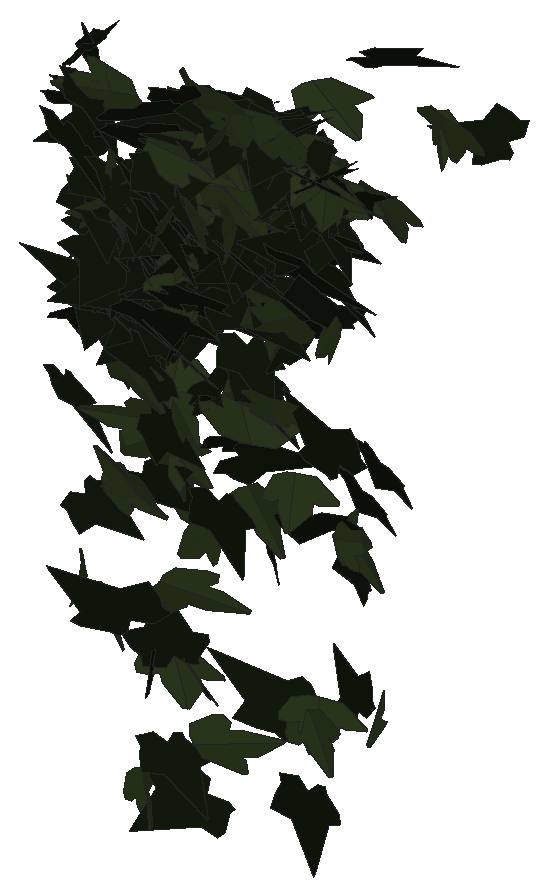
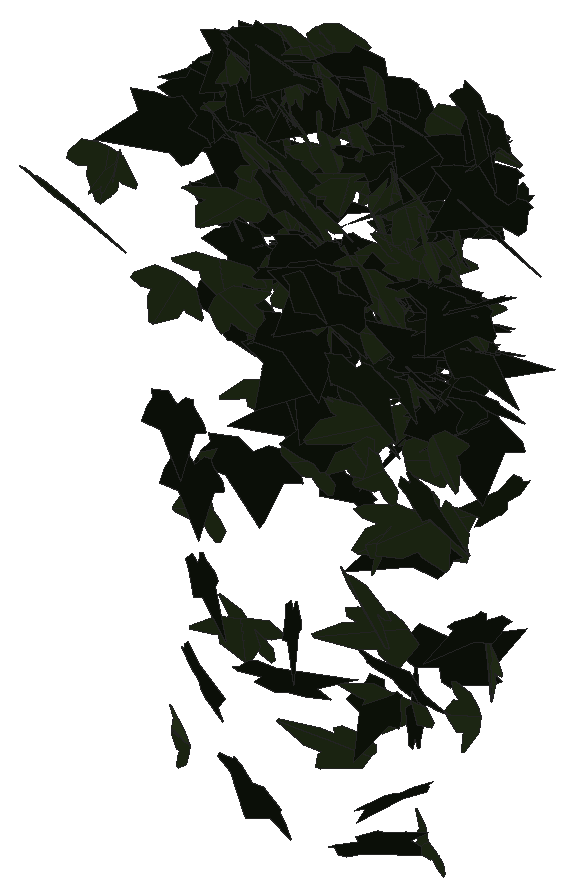
# SketchUp Ruby script. Lengths in millimetres.
U = 1.mm
M = Sketchup.active_model
def pt(a) = Geom::Point3d.new(a.map { |v| v * U })
def face(e, loops, mat)
  f = e.add_face(loops[0].map { |a| pt(a) })
  loops[1..].each { |l| e.add_face(l.map { |a| pt(a) }).erase! }
  f.material = f.back_material = mat if mat
  f
end
# faces: each face lists its corners as indices into pts; further lists are holes
def faces(e, pts, list, mat = nil) = list.each { |f| face(e, (f[0].is_a?(Array) ? f : [f]).map { |l| l.map { |i| pts[i] } }, mat) }
# xy, xz, yz: faces in a plane at the given z, y or x. An outline is a flat list of corners, or four numbers for a rectangle; further outlines are holes
def ring(l) = l.size == 4 ? [[l[0], l[1]], [l[2], l[1]], [l[2], l[3]], [l[0], l[3]]] : l.each_slice(2).to_a
def flat(e, list, mat, &to3) = list.each { |f| face(e, (f[0].is_a?(Array) ? f : [f]).map { |l| ring(l).map { |u, v| to3.(u, v) } }, mat) }
def xy(e, z, list, mat = nil) = flat(e, list, mat) { |x, y| [x, y, z] }
def xz(e, y, list, mat = nil) = flat(e, list, mat) { |x, z| [x, y, z] }
def yz(e, x, list, mat = nil) = flat(e, list, mat) { |y, z| [x, y, z] }
def lines(e, pts, list) = list.each { |a, b| e.add_line(pt(pts[a]), pt(pts[b])) }
# prism: a flat outline (further loops are holes) pulled along v
def prism(e, loops, v, mat = nil)
  f = face(e, loops, mat); d = Geom::Vector3d.new(v.map { |x| x * U })
  f.pushpull(f.normal.samedirection?(d) ? d.length : -d.length)
end
def box(e, o, s, mat = nil) = prism(e, [[o, [o[0] + s[0], o[1], o[2]], [o[0] + s[0], o[1] + s[1], o[2]], [o[0], o[1] + s[1], o[2]]]], [0, 0, s[2]], mat)
def at(x, y, z, deg = 0) = Geom::Transformation.translation(pt([x, y, z])) * Geom::Transformation.rotation(ORIGIN, Z_AXIS, deg.degrees)
def axes(o, x, y, z) = Geom::Transformation.new([*x, 0, *y, 0, *z, 0, *pt(o).to_a, 1])
def part(name) = M.definitions.add(name)
# library, detail: a bought-in or finely detailed component or shape, given as its bounding box
def library(name, o, s) = part(name).tap { |d| box(d.entities, o, s) }
def detail(e, o, s) = box(e.add_group.entities, o, s)
def put(e, d, t, mat = nil) = e.add_instance(d, t).tap { |i| i.material = mat if mat }
def group(e, t, mat = nil) = e.add_group.tap { |g| g.transformation = t; g.material = mat if mat }.entities
root = M.entities
M.materials.add("efeu1").color = [18, 25, 13]
M.materials.add("efeu2").color = [43, 57, 29]
c1 = part("ivyleaf_9")
p = [[39.1,54.8,31.7],[34.5,51.8,30.2],[-5.3,25.2,17.3],[-17.9,28.3,20.9],[-21.6,21.7,17],[-20.2,4.3,5.3],
  [-22.9,-0.3,2.5],[-17.1,-4,-0.6],[-2,-2.1,-1.2],[-0.7,-15.4,-10.1],[16.6,-22.3,-16.7],[21.1,-15.1,-12.5],
  [32.7,-10.7,-11],[46.1,-1.8,-6.6],[30.8,11.2,3.8]]
faces(c1.entities,p,[[0,1,2,3,4,5,6,7,8,9,10,11,12,13,14]],"efeu1")
c2 = part("ivyleaf_10")
p = [[0,12.8,-0.8],[-1.5,51.3,-10.9],[-4.9,51,-11.6],[-13.6,26.5,-7.3],[-13.2,15.9,-4.6],[-21.1,19.3,-7.2],
  [-29.5,16.3,-8.3],[-29.2,8.3,-6.2],[-19.7,-9.8,0.5],[-7.6,-13,4],[1,-12.2,5.8],[-0.4,51.1,-11.1],
  [-1.5,51.1,-10.9],[1,-12.4,5.9],[16.9,-12.4,3.5],[35.1,9.1,-5.1],[35,12.9,-6.1],[20.5,16.4,-4.9],
  [15.8,15,-3.8],[15.3,27.6,-7.1],[12.8,31.3,-7.8]]
faces(c2.entities,p,[[0,1,2,3,4,5,6,7,8,9,10],[11,12,0,13,14,15,16,17,18,19,20]],"efeu2")
put(root,c1,axes([4336.7,826.9,2307.8],[1.64636,0.46181,-0.34816],[-0.57705,-0.1713,-0.98057],[-0.93732,0.91661,-0.00785]))
put(root,c1,axes([4322.9,848,2418.5],[0.66586,-0.92528,0.22306],[0.13804,-0.21105,-0.9892],[1.80618,0.35724,-0.00663]))
put(root,c1,axes([4282.4,847.1,1881.3],[0.46301,0.06255,1.08971],[-2.0489,-0.17041,0.25013],[0.34267,-1.10346,0.02314]))
put(root,c2,axes([4346,845.1,2435.9],[0.56997,-0.94668,0.22063],[0.12351,-0.21088,-0.99292],[1.84587,0.30642,-0.00169]))
put(root,c1,axes([4522.6,843.7,2424.9],[1.00626,-0.4296,0.7182],[1.14423,-0.39598,-0.67945],[1.10798,0.7991,0.04941]))
put(root,c2,axes([4522.3,838.5,2360.9],[-1.30614,-0.1043,0.71245],[-1.34296,-0.09855,-0.69414],[0.27286,-0.98431,-0.00599]))
put(root,c2,axes([4379.4,838.4,2456.6],[-1.04442,0.79665,-0.17631],[0.15381,-0.15836,-0.9671],[-1.54524,-0.55422,0.0229]))
put(root,c2,axes([4531.4,843.4,2142.7],[1.04113,0.86913,-0.2398],[-0.2545,-0.19917,-1.02694],[-1.69696,0.5631,0.00689]))
put(root,c2,axes([4431.2,835.7,2580.5],[0.10633,-0.99685,-0.41769],[-0.09141,0.41555,-0.99815],[2.05498,0.07007,-0.02279]))
put(root,c2,axes([4547.5,850.1,1834.9],[1.39029,-0.29535,0.69025],[1.20953,-0.26951,-0.7879],[0.76078,0.96822,-0.00876]))
put(root,c1,axes([4415.1,850,2074.1],[-0.95308,-0.05464,-0.90576],[1.72252,0.04422,-0.50306],[0.12403,-1.03404,0.02635]))
put(root,c1,axes([4316.3,860.7,2215.4],[0.48235,-0.93383,-0.33429],[0.2204,-0.31481,0.96721],[-1.8748,-0.27727,0.0277]))
put(root,c1,axes([4184.4,857.9,2481.5],[0.57821,-0.94323,0.32201],[0.18852,-0.3064,-0.99095],[1.88748,0.31955,0.00033]))
put(root,c2,axes([4441.8,834.8,2450.9],[0.64325,-0.75033,-0.66937],[-0.24935,0.66729,-0.81415],[1.89737,0.34207,0.11993]))
put(root,c2,axes([4259.2,852.9,2048.7],[0.03094,-0.11636,1.02492],[1.92704,-0.19391,-0.03808],[0.37482,1.00654,0.11115]))
put(root,c2,axes([4300.1,842.9,2051.3],[-1.15507,0.33695,-0.68674],[-1.14276,0.33329,0.69418],[0.902,0.85374,0.00005]))
put(root,c1,axes([4334.4,853.2,2487.2],[-0.02576,-0.98001,-0.37608],[-0.01723,0.37621,-0.98001],[1.9977,-0.00939,-0.0133]))
put(root,c1,axes([4357.7,839.3,2331.6],[1.83908,0.03973,0.39257],[0.74506,0.03333,-0.967],[-0.09391,1.04248,0.01596]))
put(root,c2,axes([4444.3,839.5,2600.2],[1.07842,-0.10726,-0.85706],[-1.25103,0.6114,-0.51111],[1.06642,0.82572,0.26711]))
put(root,c2,axes([4299.9,861.3,2139.4],[-0.18622,-0.05734,-0.98275],[-1.58696,-0.52011,0.11337],[-0.99586,0.83955,0.00311]))
put(root,c2,axes([4269.8,852.1,2562.1],[-0.62328,-0.02674,0.99814],[-1.80991,-0.31185,-0.32037],[0.57928,-1.00314,0.07299]))
put(root,c1,axes([4596,837.9,2199],[0.10505,0.013,1.05977],[-1.01079,0.91869,0.01639],[-1.74558,-0.5312,0.05429]))
put(root,c2,axes([4502.7,850.6,2587.7],[-1.6085,0.20624,0.52283],[-1.06539,-0.22451,-0.81634],[-0.09559,-0.96811,0.30069]))
put(root,c1,axes([4300.5,854.9,2270.2],[1.37428,-0.63325,0.29637],[0.42664,-0.19388,-0.96043],[1.26042,0.75608,0.00195]))
put(root,c2,axes([4287.5,863,1665.3],[0.94142,-0.46315,0.75785],[1.13813,-0.4677,-0.67614],[1.2498,0.77478,0.04488]))
put(root,c2,axes([4274.9,854,2206.2],[-1.31652,0.30846,-0.60263],[0.95598,-0.34379,-0.75254],[-0.86383,-0.85057,0.08563]))
put(root,c1,axes([4432.5,855.7,2404],[1.21331,-0.69179,0.2791],[0.56068,-0.10382,-0.93022],[1.30432,0.68814,0.14024]))
put(root,c1,axes([4212.2,863.4,2545.1],[0.3497,-0.99056,0.1031],[0.0191,-0.103,-1.00742],[1.89533,0.1838,-0.00887]))
put(root,c2,axes([4338.7,848,2510.1],[0.32722,0.10037,1.09442],[1.953,0.38191,-0.19624],[-0.74881,1.03993,-0.03357]))
put(root,c1,axes([4307.3,838.8,2532.6],[1.37502,0.84775,-0.11153],[-0.14426,-0.08193,-1.11384],[-1.62094,0.72643,0.00452]))
put(root,c2,axes([4221.6,840.6,1918],[0.25639,-0.64866,-0.7827],[-0.22404,0.77428,-0.66194],[1.92169,0.17682,0.02726]))
put(root,c1,axes([4305.4,836.8,2558.9],[1.18281,0.92076,0.13104],[0.13898,0.10881,-1.11087],[-1.76458,0.62576,0.00034]))
put(root,c1,axes([4294.3,863.2,2433.9],[-1.39195,-0.05491,-0.66628],[1.27237,-0.06017,-0.72889],[-0.00014,-0.98753,0.08146]))
put(root,c1,axes([4256,858.1,2450.2],[-0.57577,-0.80343,-0.59031],[0.52539,0.52526,-0.85637],[1.82326,-0.40507,0.06036]))
put(root,c1,axes([4536.2,847.6,2451.3],[-1.14206,0.72192,0.3168],[-0.42433,0.22648,-0.93841],[-1.43917,-0.63965,0.02529]))
put(root,c1,axes([4458.1,854.8,2405.9],[-1.5319,0.56318,-0.06811],[0.12643,-0.02384,-0.98219],[-1.07222,-0.80743,-0.01851]))
put(root,c1,axes([4258.6,872.3,2295.8],[-1.38533,-0.32585,0.53966],[-0.69948,-0.45038,-0.76767],[0.97479,-0.78627,0.21608]))
put(root,c2,axes([4449.9,865.5,2085.1],[1.27779,-0.27247,0.87737],[1.55773,-0.31617,-0.72451],[0.79415,1.05858,0.00944]))
put(root,c1,axes([4539.3,862.8,2356.5],[1.49916,0.20273,0.63781],[-1.20895,-0.08367,0.8111],[0.40103,-1.01009,0.06083]))
put(root,c2,axes([4425.1,854,2545.5],[1.82145,0.15262,0.27487],[0.44638,0.23996,-0.94984],[-0.39849,0.96639,0.19244]))
put(root,c1,axes([4322.2,846.9,2158.3],[0.88214,-0.57586,-0.8525],[-0.84132,0.73282,-0.73536],[1.76798,0.63605,0.07542]))
put(root,c1,axes([4485.1,875.7,2573.5],[-1.14912,-0.78567,0.20996],[0.04773,-0.27937,-0.97327],[1.54703,-0.57497,0.18599]))
put(root,c1,axes([4482.1,868.9,2549.2],[-1.38832,-0.60821,-0.28835],[0.52732,0.11619,-0.946],[1.16749,-0.77574,0.08439]))
put(root,c2,axes([4348.4,862.3,2328.7],[1.79236,-0.18503,0.16172],[0.29742,-0.04339,-0.95969],[0.36094,0.95456,-0.01228]))
put(root,c1,axes([4389,861.7,2551.6],[-1.69256,0.28049,0.42264],[-0.81052,0.05053,-0.92966],[-0.52443,-0.98335,0.07278]))
put(root,c2,axes([4451.8,856.8,2181.7],[2.06992,0.29269,0.18353],[-0.33795,-0.04641,1.12629],[0.564,-1.102,0.00131]))
put(root,c2,axes([4459.1,864.3,2581.5],[-0.88613,-0.87306,0.18737],[-0.15134,-0.16994,-0.98941],[1.6927,-0.47225,0.00963]))
put(root,c2,axes([4272.9,849.8,2386.9],[-0.79526,0.74822,0.45618],[-0.58732,0.34737,-0.85243],[-1.56098,-0.51189,0.08832]))
put(root,c1,axes([4422.1,873.8,2573.6],[-1.2461,-0.77245,-0.08162],[0.22853,0.00481,-1.00875],[1.46054,-0.65979,0.0882]))
put(root,c1,axes([4299.4,873.3,1802.4],[0.15312,0.38579,0.9606],[-0.56981,-0.91364,0.39201],[1.88593,-0.30737,0.04045]))
put(root,c2,axes([4485.1,859.4,2224.9],[-1.8026,-0.23174,0.09144],[-0.16487,-0.03069,-0.97504],[0.44456,-0.95105,0.00919]))
put(root,c1,axes([4245.2,875.6,2329],[-1.18718,-0.71816,0.13],[-0.17645,-0.09165,-0.95119],[1.37775,-0.63056,-0.0098]))
put(root,c1,axes([4320.1,881.8,2390.7],[-1.36391,-0.52105,0.38349],[-0.152,-0.49666,-0.82406],[1.22187,-0.6434,0.32556]))
put(root,c1,axes([4252.3,863.5,2282.6],[-0.35165,0.08846,0.99512],[-1.77846,0.34265,-0.20396],[-0.67253,-0.95236,0.01905]))
put(root,c2,axes([4547.3,865,1846.2],[1.49454,0.64052,-0.09761],[-0.14355,-0.06196,-1.01338],[-1.22474,0.78889,-0.00034]))
put(root,c1,axes([4432,862,2346.9],[-0.01882,-0.55376,-0.81589],[0.93603,0.70442,-0.48407],[1.62658,-0.41177,0.26912]))
put(root,c2,axes([4540.3,881.4,2542.4],[-0.81762,-0.52454,0.73994],[0.08448,-0.82993,-0.56256],[1.72414,-0.20808,0.37846]))
put(root,c1,axes([4438.6,876.6,2416.2],[-1.1189,-0.78595,-0.12915],[0.14919,0.10264,-0.98151],[1.50853,-0.59311,0.00128]))
put(root,c2,axes([4570.4,863,2350.9],[0.89486,-0.86818,-0.31057],[-0.21441,0.29192,-0.98659],[1.74172,0.48199,0.03811]))
put(root,c1,axes([4357.2,842.6,2262.5],[0.16497,0.29612,1.08571],[0.45443,1.0593,-0.30797],[-2.09304,0.25333,0.01871]))
put(root,c1,axes([4365.8,866.2,2343.6],[-1.62969,0.46454,0.01801],[-0.02518,0.01337,-0.97417],[-0.88443,-0.85637,-0.00545]))
put(root,c2,axes([4319.4,872.4,2480.7],[1.39844,-0.64544,0.17662],[0.25266,-0.11649,-0.97801],[1.24825,0.74668,0.00009]))
put(root,c2,axes([4352.6,858.4,2171.3],[-0.25318,0.94291,0.28828],[-0.14601,0.28011,-0.95159],[-1.87085,-0.14946,0.03526]))
put(root,c1,axes([4324.8,871.5,1717],[0.20585,-0.95763,-0.34904],[-0.01574,0.35016,-0.96327],[1.93978,0.10446,0.02922]))
put(root,c2,axes([4236.4,876.2,2454.4],[0.56437,-0.85145,0.44654],[0.84624,-0.29287,-0.85371],[1.62238,0.44895,0.28996]))
put(root,c1,axes([4352.8,867.3,2510.2],[1.54418,-0.57448,-0.09652],[-0.13237,0.06878,-0.99402],[1.10074,0.81418,0.01587]))
put(root,c1,axes([4524.8,863.1,2534.4],[1.66482,-0.32857,0.32868],[0.7278,0.11076,-0.90701],[0.50266,0.92787,0.22466]))
put(root,c1,axes([4170.7,877.3,2138.1],[0.75934,-0.90696,0.08901],[0.05374,-0.08481,-0.9908],[1.73358,0.3999,-0.00827]))
put(root,c2,axes([4421.3,868.4,2471.1],[-1.69603,-0.15315,-0.37504],[0.74793,-0.10685,-0.89016],[0.18715,-0.96092,0.15876]))
put(root,c2,axes([4314.3,863.7,2444],[-1.59618,0.49111,0.21229],[-0.39179,0.06814,-0.97089],[-0.93988,-0.86245,0.04418]))
put(root,c1,axes([4360.1,882.7,2513.3],[-1.08671,-0.82078,-0.06248],[0.19118,0.006,-0.99674],[1.55492,-0.57437,0.07888]))
put(root,c1,axes([4411.1,866.2,2357.1],[0.25027,-0.39991,-0.89106],[1.21835,0.71433,-0.22612],[1.40386,-0.54864,0.35509]))
put(root,c1,axes([4356.7,854.8,2591.6],[1.49809,0.65891,0.10361],[0.16983,0.0548,-1.02642],[-1.25804,0.79204,-0.01518]))
put(root,c1,axes([4271.9,878,2444.5],[0.90465,-0.87456,0.13595],[0.18084,-0.103,-0.99481],[1.67472,0.48354,0.03398]))
put(root,c2,axes([4462.1,876.5,2565.8],[-0.08543,-0.98427,0.20514],[0.08743,-0.20714,-0.9838],[1.91151,-0.03451,0.05417]))
put(root,c2,axes([4548,873.7,2527.9],[1.90208,-0.12496,0.14333],[0.26808,-0.02865,-1.00714],[0.24313,1.00923,-0.01084]))
put(root,c1,axes([4300.4,878.4,2255.6],[-1.87327,-0.05458,-0.09049],[0.17128,0.01136,-0.98577],[0.10541,-0.98836,-0.00633]))
put(root,c2,axes([4335.9,873.3,2470.5],[-0.2608,0.94177,-0.27405],[-0.1007,-0.28341,-0.94747],[-1.86401,-0.11646,0.08953]))
put(root,c1,axes([4510.4,889.3,2509.5],[-0.42697,-0.88497,0.38336],[0.02153,-0.39598,-0.90749],[1.83539,-0.20123,0.09983]))
put(root,c1,axes([4552.8,850.6,2542.6],[0.73024,0.61781,0.68585],[0.54545,0.62631,-0.72451],[-1.67,0.47472,0.06327]))
put(root,c1,axes([4340.4,859.3,1850.3],[-1.7666,0.41046,-0.14762],[-0.27976,0.03244,1.0145],[0.78161,0.93933,0.02947]))
put(root,c2,axes([4329.8,872.5,1831.9],[1.82053,0.23973,0.27],[0.49217,0.07869,-0.98606],[-0.47957,0.99082,0.01298]))
put(root,c1,axes([4395.9,876.1,2372.1],[0.15595,0.35207,-0.91618],[-1.01845,-0.75468,-0.33787],[-1.56594,0.52589,0.1285]))
put(root,c2,axes([4528.2,882.9,2568.9],[-0.52874,-0.86274,0.42387],[0.18945,-0.46466,-0.88053],[1.81959,-0.20232,0.21485]))
put(root,c1,axes([4202.8,863,2541.9],[1.88988,0.18995,0.03398],[0.0688,-0.00816,-1.0109],[-0.36075,0.99355,-0.0148]))
put(root,c1,axes([4525.8,878.4,2577.8],[-1.88157,0.10593,-0.05742],[0.11395,0.02006,-0.99395],[-0.19899,-0.9901,-0.02628]))
put(root,c1,axes([4357.5,892.7,1655.3],[-1.37979,-0.66511,0.54562],[-0.73639,-0.38518,-0.98366],[1.46232,-0.82154,0.01947]))
put(root,c1,axes([4462.2,891.5,2369.1],[-0.77523,-0.82366,0.36064],[-0.03271,-0.38872,-0.9072],[1.71097,-0.38063,0.14606]))
put(root,c2,axes([4320.5,877.7,2371.1],[1.62868,-0.40605,0.19881],[0.3744,-0.04877,-0.94639],[0.77473,0.87719,0.03942]))
put(root,c1,axes([4532.3,886,2471.8],[-1.44187,-0.555,-0.33157],[0.61868,0.1145,-0.93442],[1.06357,-0.81902,0.09405]))
put(root,c2,axes([4391.3,867.3,1746.9],[0.65297,0.03843,-0.97279],[1.78371,0.26609,0.34106],[0.50143,-0.9966,0.05355]))
put(root,c2,axes([4384.9,879.9,2538.7],[1.29361,-0.73774,0.09596],[0.23957,-0.01406,-0.99971],[1.39547,0.6863,0.08267]))
put(root,c2,axes([4418.6,876.4,2568.2],[1.23058,-0.77001,-0.12744],[0.09858,0.20746,-0.99071],[1.48214,0.62552,0.17171]))
put(root,c2,axes([4362,871.7,2589.9],[-1.37458,0.69827,0.15516],[-0.3317,0.04206,-1.00058],[-1.32033,-0.73753,0.08984]))
put(root,c1,axes([4215.1,856.3,2596.1],[0.18988,0.79581,0.6446],[0.18008,0.63772,-0.80196],[-1.94077,0.13703,-0.01135]))
put(root,c1,axes([4541.5,890.4,2478.7],[0.24706,-0.96576,0.16948],[-0.00151,-0.17106,-0.97416],[1.86611,0.12772,-0.02322]))
put(root,c1,axes([4437.6,883.4,2236.2],[0.49656,-0.95777,-0.20472],[0.04968,0.21859,-0.98937],[1.86335,0.24941,0.08093]))
put(root,c2,axes([4210.1,889.1,1864.4],[-0.6362,0.62383,-0.84867],[0.75258,-0.75093,-0.70773],[-1.85797,-0.51778,0.00393]))
put(root,c1,axes([4443.7,858.5,2143.4],[0.19481,0.39849,-0.95616],[0.11259,0.957,0.40517],[1.96826,-0.09418,0.07146]))
put(root,c2,axes([4483.5,887.2,2324.6],[-0.27053,-0.9101,0.34763],[0.19256,-0.3632,-0.90949],[1.84413,-0.09559,0.14596]))
put(root,c2,axes([4452.5,890.7,2524.6],[0.96675,-0.56051,0.63878],[0.81475,-0.4741,-0.75643],[1.39719,0.66429,-0.00088]))
put(root,c2,axes([4261.3,883,2422.2],[1.24943,-0.72856,0.031],[0.08612,-0.00094,-0.98015],[1.38518,0.65722,0.03297]))
put(root,c1,axes([4491,877.1,2557.6],[1.65215,-0.46822,-0.09834],[-0.15109,0.05995,-0.98619],[0.89793,0.87158,0.015]))
put(root,c1,axes([4426.6,887.1,2266.7],[0.07041,-0.95839,-0.1884],[-0.04939,0.1875,-0.95892],[1.85825,0.0413,-0.01835]))
put(root,c1,axes([4537.6,887.3,2413.8],[0.88405,-0.87812,0.05848],[0.08537,-0.04242,-0.99321],[1.67277,0.46625,0.01978]))
put(root,c2,axes([4310.9,883.1,2399.3],[1.69708,0.3146,-0.20741],[-0.37969,-0.05787,-0.9455],[-0.6084,0.91367,0.01153]))
put(root,c1,axes([4225.3,865.3,2581.9],[0.14706,0.24441,-0.99432],[-1.8605,0.31424,0.00128],[0.5797,0.94652,0.25633]))
put(root,c1,axes([4246.8,886,2413.9],[1.10153,-0.79009,-0.00887],[0.0066,0.01353,-0.97934],[1.50377,0.57869,0.01079]))
put(root,c1,axes([4333.8,899.5,2276.1],[-0.41853,-0.8844,0.3419],[-0.01455,-0.34931,-0.90849],[1.80454,-0.20794,0.07197]))
put(root,c1,axes([4215.7,892.6,2264.4],[-1.52602,-0.36143,-0.36519],[0.71846,0.04477,-0.87315],[0.66337,-0.87993,0.10558]))
put(root,c2,axes([4254.8,888.2,2406.7],[-0.53918,-0.90798,0.17177],[0.12694,-0.19929,-0.94341],[1.75413,-0.26467,0.12107]))
put(root,c2,axes([4476.7,888.8,2541.2],[0.74188,-0.90322,0.13286],[0.11564,-0.11848,-0.98371],[1.73365,0.39442,0.00876]))
put(root,c1,axes([4307.5,891.3,2351.9],[-1.79593,-0.06464,-0.21251],[0.40838,-0.02559,-0.94503],[0.10925,-0.96693,0.03922]))
put(root,c1,axes([4504.7,868.2,2584.1],[0.27662,0.99306,0.14389],[0.08011,0.13923,-1.00341],[-1.90804,0.14981,-0.02127]))
put(root,c1,axes([4423.7,877.1,2547.8],[1.80654,-0.21762,-0.23757],[-0.43238,0.07196,-0.97366],[0.43476,0.97584,0.01882]))
put(root,c2,axes([4485.3,889.8,2439.7],[1.28468,-0.67362,0.27035],[0.46527,-0.13663,-0.95082],[1.30071,0.71418,0.0731]))
put(root,c1,axes([4239.5,895.6,2349.9],[-1.41722,-0.60263,-0.04579],[0.08467,0.0178,-0.95784],[1.1471,-0.74585,0.01413]))
put(root,c1,axes([4392.9,875.7,2203.2],[-0.89263,0.83705,0.12655],[-0.13675,0.10479,-0.95943],[-1.60537,-0.47435,0.01136]))
put(root,c1,axes([4544,874.7,2459.8],[1.40567,0.50277,-0.43038],[-0.73149,-0.19917,-0.89225],[-1.02541,0.8313,0.04652]))
put(root,c1,axes([4219.2,885.2,2489],[-1.6656,0.48207,0.03648],[-0.05871,0.0196,-0.99914],[-0.91822,-0.8757,-0.00228]))
put(root,c1,axes([4530.8,869.6,2548],[-0.44916,0.73124,0.63325],[-0.51019,0.57686,-0.76603],[-1.76891,-0.35206,0.06014]))
put(root,c1,axes([4296,881.9,2473.2],[0.97431,-0.72194,-0.47513],[-0.07203,0.53297,-0.85061],[1.64329,0.4514,0.24442]))
put(root,c1,axes([4340.9,876.2,1834.4],[1.43036,-0.19926,-0.68491],[-1.20194,0.27667,-0.77347],[0.63115,0.97847,0.07922]))
put(root,c2,axes([4540.2,888.3,2503.4],[1.23302,0.7063,-0.25248],[-0.42752,-0.13561,-0.95577],[-1.36202,0.68197,0.07144]))
put(root,c2,axes([4292.6,893,2353.3],[-0.3319,0.78244,-0.53018],[0.19673,-0.52011,-0.80157],[-1.78801,-0.20247,0.01022]))
put(root,c1,axes([4411,874.2,2195.2],[1.43513,0.60791,-0.08571],[-0.1113,-0.06402,-0.9685],[-1.1631,0.75621,-0.01308]))
put(root,c1,axes([4206.1,888,2253.9],[1.47083,-0.60709,0.0565],[0.07802,-0.03928,-0.98274],[1.15778,0.77389,-0.00556]))
put(root,c1,axes([4522.4,878.6,2517.7],[-0.37238,0.96299,-0.1223],[0.03004,-0.12158,-0.98263],[-1.84725,-0.1961,0.00867]))
put(root,c2,axes([4293.3,888.3,2449.4],[-0.46612,-0.9614,-0.02234],[-0.01017,0.02441,-0.99204],[1.8302,-0.24471,-0.0112]))
put(root,c1,axes([4200.3,899.5,2380.4],[-0.32394,-0.95833,0.01524],[0.03539,-0.01877,-0.97309],[1.82378,-0.16985,0.02159]))
put(root,c2,axes([4399.6,892.4,2491.7],[0.25391,-0.96725,-0.13885],[0.03231,-0.13782,0.97641],[-1.85947,-0.13448,-0.00199]))
put(root,c1,axes([4537.7,877.5,2544.1],[1.72379,0.04013,-0.61368],[-1.17012,0.08494,-0.90186],[0.0277,1.09075,0.09281]))
put(root,c1,axes([4493.7,890.1,1811.9],[-1.6303,-0.51484,-0.34167],[-0.56032,-0.1734,0.99942],[-1.03391,0.90579,-0.00287]))
put(root,c2,axes([4213.6,895.2,2370.3],[-0.62713,-0.86435,0.28217],[-0.06449,-0.28825,-0.92253],[1.72926,-0.32421,0.06793]))
put(root,c1,axes([4220.1,906.7,2280.1],[0.52651,-0.27868,-0.87738],[1.18957,-0.61575,0.39266],[-1.28631,-0.68351,0.004]))
put(root,c1,axes([4395.8,887,2129.2],[1.26068,0.73295,0.16831],[-0.21956,-0.1226,0.98792],[1.41432,-0.67236,0.00334]))
put(root,c1,axes([4240.9,904.4,2307],[-1.0998,-0.7499,0.17358],[-0.19578,-0.13987,-0.94671],[1.4518,-0.58694,0.00383]))
put(root,c2,axes([4444.6,889.4,2412],[1.61031,-0.36772,-0.35356],[-0.59114,0.17182,-0.92202],[0.77013,0.90077,0.03155]))
put(root,c2,axes([4333.3,898.2,2445.1],[0.86615,-0.80039,0.327],[0.31194,-0.28297,-0.92073],[1.6157,0.48371,0.00246]))
put(root,c1,axes([4252.2,894.4,2353.6],[0.95858,-0.8208,-0.00799],[0.08908,0.03807,-0.96116],[1.55968,0.50229,0.0598]))
put(root,c2,axes([4255.7,894.5,2408.6],[0.72014,-0.88399,-0.20248],[0.1248,-0.19215,0.96145],[-1.72146,-0.38373,-0.015]))
put(root,c2,axes([4319.5,893.8,2201.4],[0.9224,0.78049,-0.29783],[-0.31397,-0.24813,-0.91868],[-1.55859,0.51189,0.0088]))
put(root,c2,axes([4383.4,889.2,2464.8],[0.69026,0.90878,-0.04945],[-0.05156,-0.04243,-0.97843],[-1.73138,0.36357,0.00943]))
put(root,c1,axes([4179.6,876.4,2516.8],[1.63682,0.47043,0.25534],[0.37972,0.16666,-0.97907],[-0.94529,0.88152,0.04884]))
put(root,c2,axes([4328.7,881.4,1923.6],[-0.79422,-0.16365,-0.98224],[1.72042,0.38442,-0.4481],[0.79486,-0.99557,-0.01157]))
put(root,c1,axes([4327.7,900,2349.9],[0.9793,0.37373,0.736],[-1.11077,-0.44861,0.63582],[1.11097,-0.77796,-0.01307]))
put(root,c1,axes([4505.9,876.8,2337.1],[1.10843,0.79379,0.0726],[0.0642,0.06528,-0.98447],[-1.5157,0.58327,0.01139]))
put(root,c2,axes([4314.1,899.9,2339.7],[0.17693,-0.93451,0.23239],[-0.01295,-0.2341,-0.93867],[1.83268,0.08857,-0.02907]))
put(root,c1,axes([4517.2,884,2078.2],[0.90443,0.81082,-0.33488],[-0.40556,-0.26276,-0.93859],[-1.61958,0.51859,0.04803]))
put(root,c1,axes([4320.8,904.6,2280.2],[-1.55102,-0.45221,-0.25531],[0.53872,0.01149,-0.92389],[0.8286,-0.85393,0.12277]))
put(root,c1,axes([4286.2,902.6,2313.6],[0.68531,-0.89443,0.10005],[0.09176,-0.08844,-0.96412],[1.71043,0.36311,0.01164]))
put(root,c1,axes([4292.3,905.3,2262.6],[-0.71514,-0.88439,-0.09622],[0.04585,0.0943,-0.96079],[1.69248,-0.37624,-0.01463]))
put(root,c1,axes([4552.7,884.8,2479.6],[-0.98377,0.80965,0.27333],[-0.27993,0.23038,-0.96058],[-1.60208,-0.53742,0]))
put(root,c2,axes([4272.7,904.4,2253.5],[1.14496,-0.3423,0.67466],[1.10961,-0.33951,-0.69215],[0.91751,0.83775,-0.00484]))
put(root,c1,axes([4280.6,884.4,2050],[-0.0227,-0.22479,-0.93849],[0.45661,0.90841,-0.22063],[1.77899,-0.23603,0.04465]))
put(root,c2,axes([4357.4,898.2,2373.4],[-1.04902,-0.8014,0.07954],[0.09738,-0.13104,-0.96571],[1.52962,-0.54126,0.11603]))
put(root,c2,axes([4361.8,899.3,2373.9],[1.32777,-0.67705,0.08199],[0.2574,0.02239,-0.96594],[1.27219,0.7021,0.10986]))
put(root,c1,axes([4213.9,906.9,2219.8],[-0.06329,-0.9598,-0.02296],[-0.02459,0.02342,-0.96028],[1.82704,-0.03293,-0.01372]))
put(root,c2,axes([4483.6,890.4,2447.6],[-0.35193,-0.85888,0.45642],[0.16563,0.44813,0.87852],[-1.84368,0.20421,-0.0082]))
put(root,c1,axes([4243.7,902.4,2388.2],[-0.89815,-0.66497,-0.52291],[0.57627,0.42633,-0.81541],[1.50334,-0.5607,0.00016]))
put(root,c1,axes([4477.8,877.2,2589.4],[1.049,0.72166,0.43785],[-0.05314,0.53823,-0.85196],[-1.60562,0.45367,0.31426]))
put(root,c1,axes([4210.9,899.7,2331],[-0.63091,0.76712,-0.46972],[0.13155,-0.47739,-0.82844],[-1.70687,-0.32034,0.10977]))
put(root,c2,axes([4352.1,899.1,2301.6],[0.21226,-0.95978,-0.13196],[-0.00658,0.13244,-0.96617],[1.84383,0.11096,0.01175]))
put(root,c1,axes([4470.9,881.8,2468.1],[-0.02899,0.80097,0.56558],[-0.50238,0.54141,-0.77386],[-1.79724,-0.16426,0.20719]))
put(root,c2,axes([4474.9,903.1,2440.2],[-1.55468,-0.46461,0.26942],[-0.32512,-0.24017,-0.93213],[0.96907,-0.82595,0.1195]))
put(root,c2,axes([4262.5,893,2403.1],[-0.82505,-0.53228,0.70794],[0.83993,0.55357,0.68646],[-1.46155,0.6186,-0.00514]))
put(root,c1,axes([4188.7,892.5,1987.9],[0.38763,-0.42553,-0.82993],[-0.30513,0.82087,-0.46023],[1.74862,0.23757,0.10367]))
put(root,c1,axes([4471.6,905,2449],[-0.91118,0.73254,-0.44404],[0.36563,-0.40391,-0.87347],[-1.58877,-0.51307,0.05365]))
put(root,c1,axes([4559.3,887.8,2507.6],[1.06383,0.80506,0.1598],[0.21119,0.11744,-0.9798],[-1.54775,0.56938,-0.02385]))
put(root,c1,axes([4208.9,896.4,2234.6],[0.86291,0.97062,-0.41574],[-0.36136,-0.37013,-1.0712],[-1.97684,0.49134,0.01433]))
put(root,c2,axes([4340.2,908.5,2365.7],[-1.52179,-0.00173,0.54563],[-1.00996,-0.22275,-0.77836],[0.24159,-0.94205,0.18304]))
put(root,c1,axes([4490.9,916.8,1691.6],[-1.29416,0.04374,-0.95208],[1.80226,-0.10136,-0.68099],[-0.2053,-1.16558,0.02349]))
put(root,c1,axes([4324.3,900.8,2283.7],[-0.45926,0.93783,0.0854],[-0.02432,0.08489,-0.96834],[-1.7921,-0.24149,-0.00875]))
put(root,c1,axes([4373.1,897.6,2314.7],[0.49359,0.94034,0.06226],[0.02674,0.06071,-0.97544],[-1.79337,0.25971,0.00259]))
put(root,c2,axes([4274.1,907.9,2082.8],[-1.76665,-0.10382,-0.68038],[1.28828,0.06889,-0.93403],[0.2369,-1.14883,0.00548]))
put(root,c1,axes([4320.8,901.5,2283.7],[-0.73074,0.56598,0.6905],[-0.75398,0.5656,-0.68389],[-1.52279,-0.55165,0.00726]))
put(root,c1,axes([4212.8,897.3,2377.7],[1.02002,0.77957,0.25222],[0.27746,0.20585,-0.94602],[-1.53452,0.55541,-0.00339]))
put(root,c1,axes([4471.6,895.9,2263.6],[0.34003,0.59175,0.76323],[-0.1228,0.78176,-0.59101],[-1.83392,0.05737,0.18109]))
put(root,c1,axes([4247.4,905.8,2302.7],[-0.23063,-0.04696,0.95522],[1.72721,0.29812,0.12979],[-0.57423,0.91556,0.00673]))
put(root,c2,axes([4560.3,897.6,2055.9],[-0.26989,0.44389,0.94563],[-0.44308,0.91687,-0.46531],[-1.93813,-0.27142,-0.02531]))
put(root,c2,axes([4341.9,919.8,1989.1],[1.43569,-0.82872,-0.33081],[-0.43669,0.23847,-1.1206],[1.64114,0.78843,-0.00878]))
put(root,c1,axes([4406.1,913.2,2383],[0.52432,0.85003,-0.3728],[-0.31509,-0.33764,-0.8922],[-1.73821,0.31761,0.04928]))
put(root,c2,axes([4318.2,901.7,2045.6],[0.16711,0.40548,-0.90284],[0.19068,0.89809,0.41309],[1.87396,-0.12754,0.03847]))
put(root,c2,axes([4326.1,927.1,2314.8],[-0.80104,0.02648,-0.86094],[1.50637,-0.36613,-0.3982],[-0.6467,-0.88562,0.13888]))
put(root,c2,axes([4532.2,942,2030],[0.93384,-0.38603,0.86918],[1.5737,-0.31005,-0.60449],[0.89425,0.94874,0.15611]))
put(root,c2,axes([4202.9,949.7,2225.2],[-0.04889,-0.94211,0.10099],[0.00042,-0.10103,-0.94246],[1.8033,-0.02552,0.00296]))
put(root,c1,axes([4575.3,943.3,2142.5],[1.10216,0.00624,-0.82687],[-1.56287,0.12282,-0.5742],[0.1847,1.002,0.07554]))
put(root,c1,axes([4543.6,941.3,1812.9],[-0.04312,0.18044,1.03554],[-0.30631,1.02297,-0.18177],[-1.97694,-0.16244,0.00558]))
put(root,c1,axes([4538.4,957.5,2087],[1.07426,0.06045,-0.83067],[-1.5762,0.14705,-0.55206],[0.16795,0.99348,0.13226]))
put(root,c1,axes([4223.1,970.7,2178.1],[-1.10332,0.70231,-0.26845],[0.27813,-0.22727,-0.91015],[-1.40367,-0.59707,0.03067]))
put(root,c1,axes([4389.6,973.1,1962.7],[0.54477,-0.09926,-0.94411],[-1.59829,0.43334,-0.30017],[0.84248,0.88628,0.04103]))
put(root,c1,axes([4516.4,975.6,1977.8],[0.34932,-0.04758,-0.98882],[-1.81767,0.25616,-0.1896],[0.49586,0.97254,0.00156]))
put(root,c2,axes([4535,982.3,1756.4],[0.7354,-0.63857,0.67365],[-0.61916,0.59023,0.7461],[-1.6545,-0.50471,0.02021]))
put(root,c2,axes([4434.9,1040.4,2410],[1.80239,0.25315,-0.02818],[-0.0738,0.03606,-0.97926],[-0.47913,0.94676,0.04483]))
put(root,c1,axes([4324.3,1062.9,2456.2],[-1.15279,-0.75027,0.13069],[-0.19432,-0.08547,-0.96392],[1.43634,-0.61373,-0.02552]))
put(root,c2,axes([4296.1,1063.7,2437],[-1.38198,-0.64271,0.01976],[-0.03391,-0.00969,-0.96971],[1.22332,-0.72634,-0.00455]))
put(root,c2,axes([4276.6,1051,2385.8],[-0.58936,0.6152,0.70883],[-0.9327,0.5306,-0.67461],[-1.52345,-0.56285,0.1388]))
put(root,c1,axes([4283.8,1061.7,2449.1],[-0.31432,0.90966,-0.30338],[-0.16197,-0.32053,-0.91477],[-1.81781,-0.12873,0.13396]))
put(root,c2,axes([4396.2,1060.7,2512.6],[1.21647,0.58498,0.50192],[0.74908,0.31292,-0.86593],[-1.26131,0.75003,-0.03019]))
put(root,c1,axes([4311.7,1082.4,2397.8],[0.34809,-0.94512,-0.01882],[0.13947,0.03329,-0.95947],[1.79369,0.18083,0.07826]))
put(root,c2,axes([4384.6,1088.7,2402.7],[-0.55727,-0.72583,0.57557],[-0.15129,-0.58172,-0.77403],[1.75651,-0.28038,0.11594]))
put(root,c1,axes([4257.1,1065.6,2449.7],[1.72264,0.36895,0.04233],[0.07296,0.01809,-0.97743],[-0.70302,0.90594,0.00228]))
put(root,c2,axes([4209.2,1069.7,2302.6],[0.91846,0.11114,0.84976],[0.92695,0.76686,-0.37689],[-1.34204,0.60573,0.32124]))
put(root,c1,axes([4466.1,1066.6,2583.3],[1.35129,0.32048,0.63042],[0.96477,0.39226,-0.77033],[-0.9385,0.86468,0.1158]))
put(root,c2,axes([4173.5,1090.3,2265],[1.04627,-0.43926,0.63584],[1.2273,-0.1693,-0.6745],[0.81059,0.82331,0.20054]))
put(root,c2,axes([4470,1080.5,2391.4],[-1.75602,0.37899,-0.11821],[0.21727,-0.03317,-0.99739],[-0.72365,-0.92962,-0.01261]))
put(root,c1,axes([4293.1,1075.2,2395.6],[0.59012,0.86617,-0.28105],[-0.26007,-0.24928,-0.91901],[-1.71348,0.33614,0.04269]))
put(root,c2,axes([4209.5,1089.6,2279.5],[0.58942,0.78323,-0.43615],[-0.57393,-0.34354,-0.83104],[-1.60675,0.41003,0.13685]))
put(root,c2,axes([4548.4,1089,2514.8],[-0.03878,0.94308,-0.29113],[-0.11537,-0.29184,-0.94114],[-1.87491,-0.00155,0.06393]))
put(root,c1,axes([4293.5,1070.3,2354.2],[1.30293,0.68212,0.23219],[0.29577,0.17296,-0.96634],[-1.33908,0.70191,0.01248]))
put(root,c1,axes([4216.5,1075.2,2370.7],[-0.18942,0.94835,0.08723],[-0.33547,0.06785,-0.93873],[-1.78121,-0.11363,0.16752]))
put(root,c2,axes([4563.4,1084.1,2519.3],[-1.74021,0.36362,0.11866],[-0.23992,0.00381,-0.98308],[-0.68728,-0.92202,0.04274]))
put(root,c1,axes([4605.7,1132.4,2492.8],[-1.1395,0.74006,0.36971],[-0.66596,0.187,-0.94098],[-1.4267,-0.67838,0.14394]))
